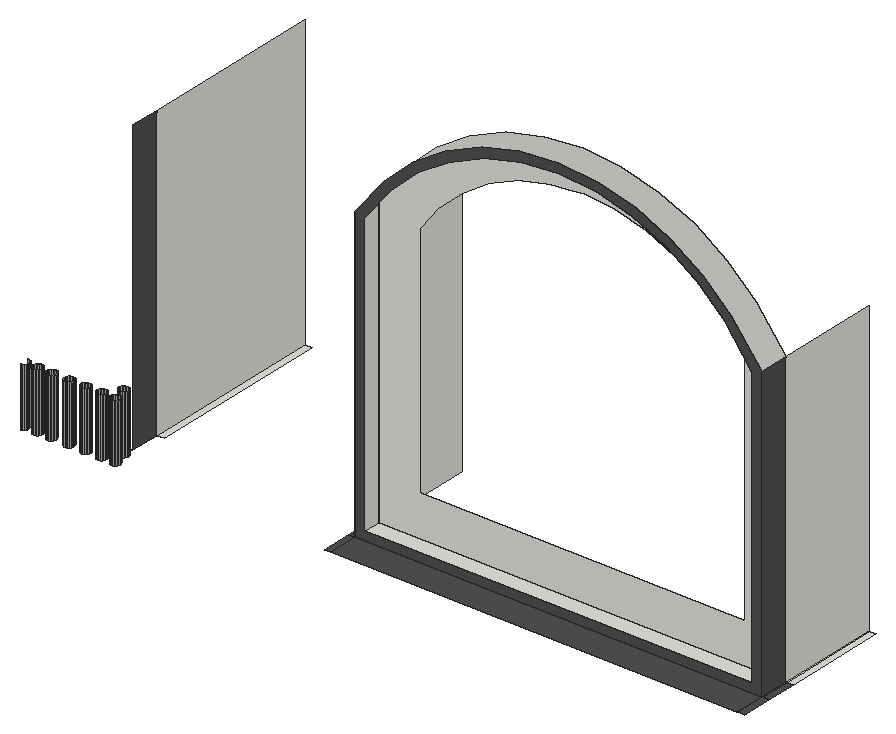
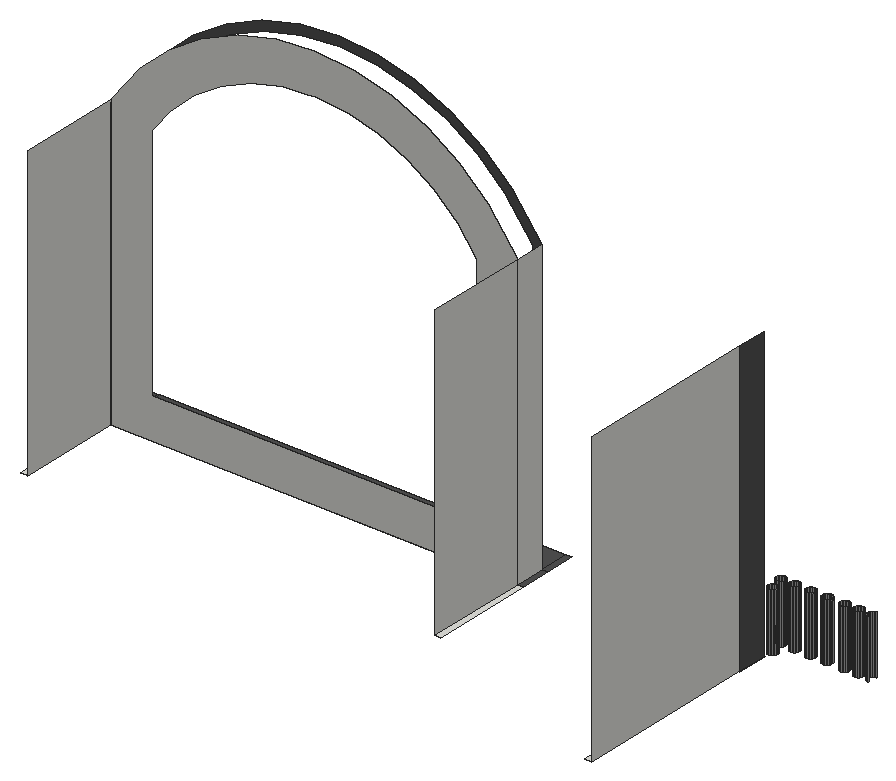
# SketchUp Ruby script. Lengths in inches.
U = 1.inch
M = Sketchup.active_model
def pt(a) = Geom::Point3d.new(a.map { |v| v * U })
def face(e, loops, mat)
  f = e.add_face(loops[0].map { |a| pt(a) })
  loops[1..].each { |l| e.add_face(l.map { |a| pt(a) }).erase! }
  f.material = f.back_material = mat if mat
  f
end
# faces: each face lists its corners as indices into pts; further lists are holes
def faces(e, pts, list, mat = nil) = list.each { |f| face(e, (f[0].is_a?(Array) ? f : [f]).map { |l| l.map { |i| pts[i] } }, mat) }
# xy, xz, yz: faces in a plane at the given z, y or x. An outline is a flat list of corners, or four numbers for a rectangle; further outlines are holes
def ring(l) = l.size == 4 ? [[l[0], l[1]], [l[2], l[1]], [l[2], l[3]], [l[0], l[3]]] : l.each_slice(2).to_a
def flat(e, list, mat, &to3) = list.each { |f| face(e, (f[0].is_a?(Array) ? f : [f]).map { |l| ring(l).map { |u, v| to3.(u, v) } }, mat) }
def xy(e, z, list, mat = nil) = flat(e, list, mat) { |x, y| [x, y, z] }
def xz(e, y, list, mat = nil) = flat(e, list, mat) { |x, z| [x, y, z] }
def yz(e, x, list, mat = nil) = flat(e, list, mat) { |y, z| [x, y, z] }
def lines(e, pts, list) = list.each { |a, b| e.add_line(pt(pts[a]), pt(pts[b])) }
# prism: a flat outline (further loops are holes) pulled along v
def prism(e, loops, v, mat = nil)
  f = face(e, loops, mat); d = Geom::Vector3d.new(v.map { |x| x * U })
  f.pushpull(f.normal.samedirection?(d) ? d.length : -d.length)
end
def box(e, o, s, mat = nil) = prism(e, [[o, [o[0] + s[0], o[1], o[2]], [o[0] + s[0], o[1] + s[1], o[2]], [o[0], o[1] + s[1], o[2]]]], [0, 0, s[2]], mat)
def at(x, y, z, deg = 0) = Geom::Transformation.translation(pt([x, y, z])) * Geom::Transformation.rotation(ORIGIN, Z_AXIS, deg.degrees)
def axes(o, x, y, z) = Geom::Transformation.new([*x, 0, *y, 0, *z, 0, *pt(o).to_a, 1])
def part(name) = M.definitions.add(name)
# library, detail: a bought-in or finely detailed component or shape, given as its bounding box
def library(name, o, s) = part(name).tap { |d| box(d.entities, o, s) }
def detail(e, o, s) = box(e.add_group.entities, o, s)
def put(e, d, t, mat = nil) = e.add_instance(d, t).tap { |i| i.material = mat if mat }
def group(e, t, mat = nil) = e.add_group.tap { |g| g.transformation = t; g.material = mat if mat }.entities
root = M.entities
M.materials.add("[0132_LightGray]").color = [169, 169, 169]
M.materials.add("[0135_DarkGray]").color = [81, 81, 81]
xy(root,180.28,[[338.62,32.09,338.25,32.13,337.9,32.28,337.6,32.51,337.375,32.8,337.23,33.15,337.18,33.52,337.23,33.89,337.375,34.24,337.6,34.54,337.9,34.77,338.25,34.91,338.62,34.96,338.99,34.91,339.34,34.77,339.64,34.54,339.87,34.24,340.01,33.89,340.06,33.52,340.01,33.15,339.87,32.8,339.64,32.51,339.34,32.28,338.99,32.13],[342.68,32.09,342.3125,32.13,341.97,32.28,341.67,32.51,341.4375,32.8,341.3,33.15,341.25,33.52,341.3,33.89,341.4375,34.24,341.67,34.54,341.97,34.77,342.3125,34.91,342.68,34.96,343.06,34.91,343.4,34.77,343.7,34.54,343.93,34.24,344.07,33.89,344.12,33.52,344.07,33.15,343.93,32.8,343.7,32.51,343.4,32.28,343.06,32.13],[347.93,32.09,347.5625,32.13,347.22,32.28,346.92,32.51,346.6875,32.8,346.55,33.15,346.5,33.52,346.55,33.89,346.6875,34.24,346.92,34.54,347.22,34.77,347.5625,34.91,347.93,34.96,348.31,34.91,348.65,34.77,348.95,34.54,349.18,34.24,349.32,33.89,349.37,33.52,349.32,33.15,349.18,32.8,348.95,32.51,348.65,32.28,348.31,32.13],[352.81,32.09,352.4375,32.13,352.09,32.28,351.79,32.51,351.5625,32.8,351.42,33.15,351.37,33.52,351.42,33.89,351.5625,34.24,351.79,34.54,352.09,34.77,352.4375,34.91,352.81,34.96,353.18,34.91,353.53,34.77,353.83,34.54,354.05,34.24,354.2,33.89,354.25,33.52,354.2,33.15,354.05,32.8,353.83,32.51,353.53,32.28,353.18,32.13],[357.56,32.09,357.1875,32.13,356.84,32.28,356.54,32.51,356.3125,32.8,356.17,33.15,356.12,33.52,356.17,33.89,356.3125,34.24,356.54,34.54,356.84,34.77,357.1875,34.91,357.56,34.96,357.93,34.91,358.28,34.77,358.58,34.54,358.8,34.24,358.95,33.89,359,33.52,358.95,33.15,358.8,32.8,358.58,32.51,358.28,32.28,357.93,32.13],
  [361.68,32.09,361.3125,32.13,360.97,32.28,360.67,32.51,360.4375,32.8,360.3,33.15,360.25,33.52,360.3,33.89,360.4375,34.24,360.67,34.54,360.97,34.77,361.3125,34.91,361.68,34.96,362.06,34.91,362.4,34.77,362.7,34.54,362.93,34.24,363.07,33.89,363.12,33.52,363.07,33.15,362.93,32.8,362.7,32.51,362.4,32.28,362.06,32.13],[360.7,36.35,360.32,36.4,359.98,36.54,359.68,36.77,359.45,37.07,359.31,37.41,359.26,37.78,359.31,38.16,359.45,38.5,359.68,38.8,359.98,39.03,360.32,39.17,360.7,39.22,361.07,39.17,361.41,39.03,361.71,38.8,361.94,38.5,362.08,38.16,362.13,37.78,362.08,37.41,361.94,37.07,361.71,36.77,361.41,36.54,361.07,36.4],[360.89,40.6875,361.14,49.6875],[426.95,40.6875,547.64,49.6875],[361.14,49.6875,363.26,104.375],
  [425.2,49.6875,426.95,80.4375],[547.64,49.6875,548.14,80.4375],[548.14,49.6875,549.95,80.4375]])
xy(root,180.28,[[425.2,31.6875,426.95,40.6875],[426.95,31.6875,547.64,40.6875],[547.64,31.6875,548.14,40.6875],[548.14,31.6875,549.95,40.6875],[425.2,40.6875,426.95,49.6875],
  [547.64,40.6875,548.14,49.6875],[548.14,40.6875,549.95,49.6875]],"[0135_DarkGray]")
xz(root,40.6875,[[[426.95,180.28,547.64,180.28,547.64,266.7,538.71,278.3,530.24,286.17,520.59,292.53,510.01,297.2,498.8125,300.05,487.29,301.01,475.77,300.05,464.57,297.2,454,292.53,444.34,286.17,435.875,278.3,426.95,266.7],[429.64,182.98,429.64,265.78,437.875,276.48,446.01,284.04,455.29,290.15,465.45,294.64,476.22,297.38,487.29,298.31,498.36,297.38,509.13,294.64,519.29,290.15,528.57,284.04,536.71,276.48,544.9375,265.78,544.9375,182.98]]],"[0135_DarkGray]")
xz(root,49.6875,[[[426.95,180.28,426.95,266.7,435.875,278.3,444.34,286.17,454,292.53,464.57,297.2,475.77,300.05,487.29,301.01,498.8125,300.05,510.01,297.2,520.59,292.53,530.24,286.17,538.71,278.3,547.64,266.7,547.64,180.28],[438.95,192.28,535.64,192.28,535.64,262.62,529.81,270.19,522.8,276.7,514.82,281.95,506.08,285.82,496.82,288.18,489.7,288.77,487.29,288.97,483.7,288.67,477.77,288.18,468.5,285.82,459.76,281.95,451.78,276.7,444.78,270.19,438.95,262.62]]])
yz(root,361.14,[[49.6875,180.28,104.375,266.7]])
yz(root,361.14,[[40.6875,180.28,49.6875,266.7]],"[0135_DarkGray]")
yz(root,426.95,[[40.6875,180.28,49.6875,266.7],[49.6875,180.28,80.4375,266.7]])
yz(root,547.64,[[49.6875,180.28,80.4375,266.7]])
yz(root,547.64,[[40.6875,180.28,49.6875,266.7]],"[0135_DarkGray]")
p = [[334.56,32.09,180.28],[334.93,32.13,180.28],[334.93,32.13,197.66],[334.56,32.09,197.66],[335.28,32.28,180.28],[335.28,32.28,197.66],
  [337.9,32.28,180.28],[338.25,32.13,180.28],[338.25,32.13,197.66],[337.9,32.28,197.66],[338.62,32.09,180.28],[338.62,32.09,197.66],
  [338.99,32.13,180.28],[338.99,32.13,197.66],[339.34,32.28,180.28],[339.34,32.28,197.66],[341.97,32.28,180.28],[342.3125,32.13,180.28],
  [342.3125,32.13,197.66],[341.97,32.28,197.66],[342.68,32.09,180.28],[342.68,32.09,197.66],[343.06,32.13,180.28],[343.06,32.13,197.66],
  [343.4,32.28,180.28],[343.4,32.28,197.66],[347.22,32.28,180.28],[347.5625,32.13,180.28],[347.5625,32.13,197.66],[347.22,32.28,197.66],
  [347.93,32.09,180.28],[347.93,32.09,197.66],[348.31,32.13,180.28],[348.31,32.13,197.66],[348.65,32.28,180.28],[348.65,32.28,197.66],
  [352.09,32.28,180.28],[352.4375,32.13,180.28],[352.4375,32.13,197.66],[352.09,32.28,197.66],[352.81,32.09,180.28],[352.81,32.09,197.66],
  [353.18,32.13,180.28],[353.18,32.13,197.66],[353.53,32.28,180.28],[353.53,32.28,197.66],[356.84,32.28,180.28],[357.1875,32.13,180.28],
  [357.1875,32.13,197.66],[356.84,32.28,197.66],[357.56,32.09,180.28],[357.56,32.09,197.66],[357.93,32.13,180.28],[357.93,32.13,197.66],
  [358.28,32.28,180.28],[358.28,32.28,197.66],[360.97,32.28,180.28],[361.3125,32.13,180.28],[361.3125,32.13,197.66],[360.97,32.28,197.66],
  [361.68,32.09,180.28],[361.68,32.09,197.66],[362.06,32.13,180.28],[362.06,32.13,197.66],[362.4,32.28,180.28],[362.4,32.28,197.66],
  [335.58,32.51,180.28],[335.58,32.51,197.66],[337.6,32.51,180.28],[337.6,32.51,197.66],[339.64,32.51,180.28],[339.64,32.51,197.66],
  [341.67,32.51,180.28],[341.67,32.51,197.66],[343.7,32.51,180.28],[343.7,32.51,197.66],[346.92,32.51,180.28],[346.92,32.51,197.66],
  [348.95,32.51,180.28],[348.95,32.51,197.66],[351.79,32.51,180.28],[351.79,32.51,197.66],[353.83,32.51,180.28],[353.83,32.51,197.66],
  [356.54,32.51,180.28],[356.54,32.51,197.66],[358.58,32.51,180.28],[358.58,32.51,197.66],[360.67,32.51,180.28],[360.67,32.51,197.66],
  [362.7,32.51,180.28],[362.7,32.51,197.66],[335.8,32.8,180.28],[335.8,32.8,197.66],[337.375,32.8,180.28],[337.375,32.8,197.66],
  [339.87,32.8,180.28],[339.87,32.8,197.66],[341.4375,32.8,180.28],[341.4375,32.8,197.66],[343.93,32.8,180.28],[343.93,32.8,197.66],
  [346.6875,32.8,180.28],[346.6875,32.8,197.66],[349.18,32.8,180.28],[349.18,32.8,197.66],[351.5625,32.8,180.28],[351.5625,32.8,197.66],
  [354.05,32.8,180.28],[354.05,32.8,197.66],[356.3125,32.8,180.28],[356.3125,32.8,197.66],[358.8,32.8,180.28],[358.8,32.8,197.66],
  [360.4375,32.8,180.28],[360.4375,32.8,197.66],[362.93,32.8,180.28],[362.93,32.8,197.66],[335.95,33.15,180.28],[335.95,33.15,197.66],
  [337.23,33.15,180.28],[337.23,33.15,197.66],[340.01,33.15,180.28],[340.01,33.15,197.66],[341.3,33.15,180.28],[341.3,33.15,197.66],
  [344.07,33.15,180.28],[344.07,33.15,197.66],[346.55,33.15,180.28],[346.55,33.15,197.66],[349.32,33.15,180.28],[349.32,33.15,197.66],
  [351.42,33.15,180.28],[351.42,33.15,197.66],[354.2,33.15,180.28],[354.2,33.15,197.66],[356.17,33.15,180.28],[356.17,33.15,197.66],
  [358.95,33.15,180.28],[358.95,33.15,197.66],[360.3,33.15,180.28],[360.3,33.15,197.66],[363.07,33.15,180.28],[363.07,33.15,197.66],
  [336,33.52,180.28],[336,33.52,197.66],[337.18,33.52,180.28],[337.18,33.52,197.66],[340.06,33.52,180.28],[340.06,33.52,197.66],
  [341.25,33.52,180.28],[341.25,33.52,197.66],[344.12,33.52,180.28],[344.12,33.52,197.66],[346.5,33.52,180.28],[346.5,33.52,197.66],
  [349.37,33.52,180.28],[349.37,33.52,197.66],[351.37,33.52,180.28],[351.37,33.52,197.66],[354.25,33.52,180.28],[354.25,33.52,197.66],
  [356.12,33.52,180.28],[356.12,33.52,197.66],[359,33.52,180.28],[359,33.52,197.66],[360.25,33.52,180.28],[360.25,33.52,197.66],
  [363.12,33.52,180.28],[363.12,33.52,197.66],[335.95,33.89,180.28],[335.95,33.89,197.66],[337.23,33.89,180.28],[337.23,33.89,197.66],
  [340.01,33.89,180.28],[340.01,33.89,197.66],[341.3,33.89,180.28],[341.3,33.89,197.66],[344.07,33.89,180.28],[344.07,33.89,197.66],
  [346.55,33.89,180.28],[346.55,33.89,197.66],[349.32,33.89,180.28],[349.32,33.89,197.66],[351.42,33.89,180.28],[351.42,33.89,197.66],
  [354.2,33.89,180.28],[354.2,33.89,197.66],[356.17,33.89,180.28],[356.17,33.89,197.66],[358.95,33.89,180.28],[358.95,33.89,197.66],
  [360.3,33.89,180.28],[360.3,33.89,197.66],[363.07,33.89,180.28],[363.07,33.89,197.66],[335.8,34.24,180.28],[335.8,34.24,197.66],
  [337.375,34.24,180.28],[337.375,34.24,197.66],[339.87,34.24,180.28],[339.87,34.24,197.66],[341.4375,34.24,180.28],[341.4375,34.24,197.66],
  [343.93,34.24,180.28],[343.93,34.24,197.66],[346.6875,34.24,180.28],[346.6875,34.24,197.66],[349.18,34.24,180.28],[349.18,34.24,197.66],
  [351.5625,34.24,180.28],[351.5625,34.24,197.66],[354.05,34.24,180.28],[354.05,34.24,197.66],[356.3125,34.24,180.28],[356.3125,34.24,197.66],
  [358.8,34.24,180.28],[358.8,34.24,197.66],[360.4375,34.24,180.28],[360.4375,34.24,197.66],[362.93,34.24,180.28],[362.93,34.24,197.66],
  [335.58,34.54,180.28],[335.58,34.54,197.66],[337.6,34.54,180.28],[337.6,34.54,197.66],[339.64,34.54,180.28],[339.64,34.54,197.66],
  [341.67,34.54,180.28],[341.67,34.54,197.66],[343.7,34.54,180.28],[343.7,34.54,197.66],[346.92,34.54,180.28],[346.92,34.54,197.66],
  [348.95,34.54,180.28],[348.95,34.54,197.66],[351.79,34.54,180.28],[351.79,34.54,197.66],[353.83,34.54,180.28],[353.83,34.54,197.66],
  [356.54,34.54,180.28],[356.54,34.54,197.66],[358.58,34.54,180.28],[358.58,34.54,197.66],[360.67,34.54,180.28],[360.67,34.54,197.66],
  [362.7,34.54,180.28],[362.7,34.54,197.66],[335.28,34.77,180.28],[335.28,34.77,197.66],[337.9,34.77,180.28],[337.9,34.77,197.66],
  [339.34,34.77,180.28],[339.34,34.77,197.66],[341.97,34.77,180.28],[341.97,34.77,197.66],[343.4,34.77,180.28],[343.4,34.77,197.66],
  [347.22,34.77,180.28],[347.22,34.77,197.66],[348.65,34.77,180.28],[348.65,34.77,197.66],[352.09,34.77,180.28],[352.09,34.77,197.66],
  [353.53,34.77,180.28],[353.53,34.77,197.66],[356.84,34.77,180.28],[356.84,34.77,197.66],[358.28,34.77,180.28],[358.28,34.77,197.66],
  [360.97,34.77,180.28],[360.97,34.77,197.66],[362.4,34.77,180.28],[362.4,34.77,197.66],[334.93,34.91,180.28],[334.93,34.91,197.66],
  [338.25,34.91,180.28],[338.25,34.91,197.66],[338.99,34.91,180.28],[338.99,34.91,197.66],[342.3125,34.91,180.28],[342.3125,34.91,197.66],
  [343.06,34.91,180.28],[343.06,34.91,197.66],[347.5625,34.91,180.28],[347.5625,34.91,197.66],[348.31,34.91,180.28],[348.31,34.91,197.66],
  [352.4375,34.91,180.28],[352.4375,34.91,197.66],[353.18,34.91,180.28],[353.18,34.91,197.66],[357.1875,34.91,180.28],[357.1875,34.91,197.66],
  [357.93,34.91,180.28],[357.93,34.91,197.66],[361.3125,34.91,180.28],[361.3125,34.91,197.66],[362.06,34.91,180.28],[362.06,34.91,197.66],
  [334.56,34.96,180.28],[334.56,34.96,197.66],[338.62,34.96,180.28],[338.62,34.96,197.66],[342.68,34.96,180.28],[342.68,34.96,197.66],
  [347.93,34.96,180.28],[347.93,34.96,197.66],[352.81,34.96,180.28],[352.81,34.96,197.66],[357.56,34.96,180.28],[357.56,34.96,197.66],
  [361.68,34.96,180.28],[361.68,34.96,197.66],[360.32,36.4,180.28],[360.7,36.35,180.28],[360.7,36.35,197.66],[360.32,36.4,197.66],
  [361.07,36.4,180.28],[361.07,36.4,197.66],[359.98,36.54,180.28],[359.98,36.54,197.66],[361.41,36.54,180.28],[361.41,36.54,197.66],
  [359.68,36.77,180.28],[359.68,36.77,197.66],[361.71,36.77,180.28],[361.71,36.77,197.66],[359.45,37.07,180.28],[359.45,37.07,197.66],
  [361.94,37.07,180.28],[361.94,37.07,197.66],[359.31,37.41,180.28],[359.31,37.41,197.66],[362.08,37.41,180.28],[362.08,37.41,197.66],
  [359.26,37.78,180.28],[359.26,37.78,197.66],[362.13,37.78,180.28],[362.13,37.78,197.66],[359.31,38.16,180.28],[359.31,38.16,197.66],
  [362.08,38.16,180.28],[362.08,38.16,197.66],[359.45,38.5,180.28],[359.45,38.5,197.66],[361.94,38.5,180.28],[361.94,38.5,197.66],
  [359.68,38.8,180.28],[359.68,38.8,197.66],[361.71,38.8,180.28],[361.71,38.8,197.66],[359.98,39.03,180.28],[359.98,39.03,197.66],
  [361.41,39.03,180.28],[361.41,39.03,197.66],[360.32,39.17,180.28],[360.32,39.17,197.66],[361.07,39.17,180.28],[361.07,39.17,197.66],
  [360.7,39.22,180.28],[360.7,39.22,197.66]]
faces(root,p,[[0,1,2,3],[1,4,5,2],[6,7,8,9],[7,10,11,8],[10,12,13,11],[12,14,15,13],[16,17,18,19],[17,20,21,18],
  [20,22,23,21],[22,24,25,23],[26,27,28,29],[27,30,31,28],[30,32,33,31],[32,34,35,33],[36,37,38,39],[37,40,41,38],
  [40,42,43,41],[42,44,45,43],[46,47,48,49],[47,50,51,48],[50,52,53,51],[52,54,55,53],[56,57,58,59],[57,60,61,58],
  [60,62,63,61],[62,64,65,63],[4,66,67,5],[68,6,9,69],[14,70,71,15],[72,16,19,73],[24,74,75,25],[76,26,29,77],
  [34,78,79,35],[80,36,39,81],[44,82,83,45],[84,46,49,85],[54,86,87,55],[88,56,59,89],[64,90,91,65],[66,92,93,67],
  [94,68,69,95],[70,96,97,71],[98,72,73,99],[74,100,101,75],[102,76,77,103],[78,104,105,79],[106,80,81,107],[82,108,109,83],
  [110,84,85,111],[86,112,113,87],[114,88,89,115],[90,116,117,91],[92,118,119,93],[120,94,95,121],[96,122,123,97],[124,98,99,125],
  [100,126,127,101],[128,102,103,129],[104,130,131,105],[132,106,107,133],[108,134,135,109],[136,110,111,137],[112,138,139,113],[140,114,115,141],
  [116,142,143,117],[118,144,145,119],[146,120,121,147],[122,148,149,123],[150,124,125,151],[126,152,153,127],[154,128,129,155],[130,156,157,131],
  [158,132,133,159],[134,160,161,135],[162,136,137,163],[138,164,165,139],[166,140,141,167],[142,168,169,143],[144,170,171,145],[172,146,147,173],
  [148,174,175,149],[176,150,151,177],[152,178,179,153],[180,154,155,181],[156,182,183,157],[184,158,159,185],[160,186,187,161],[188,162,163,189],
  [164,190,191,165],[192,166,167,193],[168,194,195,169],[170,196,197,171],[198,172,173,199],[174,200,201,175],[202,176,177,203],[178,204,205,179],
  [206,180,181,207],[182,208,209,183],[210,184,185,211],[186,212,213,187],[214,188,189,215],[190,216,217,191],[218,192,193,219],[194,220,221,195],
  [196,222,223,197],[224,198,199,225],[200,226,227,201],[228,202,203,229],[204,230,231,205],[232,206,207,233],[208,234,235,209],[236,210,211,237],
  [212,238,239,213],[240,214,215,241],[216,242,243,217],[244,218,219,245],[220,246,247,221],[222,248,249,223],[250,224,225,251],[226,252,253,227],
  [254,228,229,255],[230,256,257,231],[258,232,233,259],[234,260,261,235],[262,236,237,263],[238,264,265,239],[266,240,241,267],[242,268,269,243],
  [270,244,245,271],[246,272,273,247],[248,274,275,249],[276,250,251,277],[252,278,279,253],[280,254,255,281],[256,282,283,257],[284,258,259,285],
  [260,286,287,261],[288,262,263,289],[264,290,291,265],[292,266,267,293],[268,294,295,269],[296,270,271,297],[272,298,299,273],[274,300,301,275],
  [302,276,277,303],[278,302,303,279],[304,280,281,305],[282,304,305,283],[306,284,285,307],[286,306,307,287],[308,288,289,309],[290,308,309,291],
  [310,292,293,311],[294,310,311,295],[312,296,297,313],[298,312,313,299],[314,315,316,317],[315,318,319,316],[320,314,317,321],[318,322,323,319],
  [324,320,321,325],[322,326,327,323],[328,324,325,329],[326,330,331,327],[332,328,329,333],[330,334,335,331],[336,332,333,337],[334,338,339,335],
  [340,336,337,341],[338,342,343,339],[344,340,341,345],[342,346,347,343],[348,344,345,349],[346,350,351,347],[352,348,349,353],[350,354,355,351],
  [356,352,353,357],[354,358,359,355],[360,356,357,361],[358,360,361,359]],"[0132_LightGray]")
